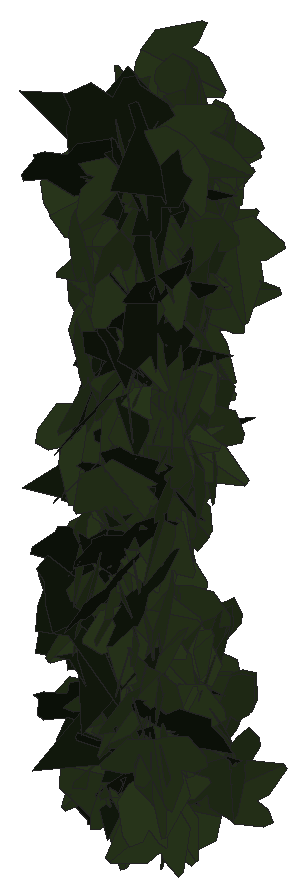
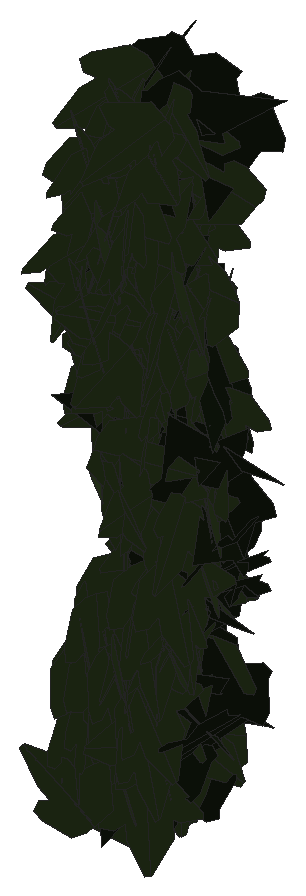
# SketchUp Ruby script. Lengths in inches.
U = 1.inch
M = Sketchup.active_model
def pt(a) = Geom::Point3d.new(a.map { |v| v * U })
def face(e, loops, mat)
  f = e.add_face(loops[0].map { |a| pt(a) })
  loops[1..].each { |l| e.add_face(l.map { |a| pt(a) }).erase! }
  f.material = f.back_material = mat if mat
  f
end
# faces: each face lists its corners as indices into pts; further lists are holes
def faces(e, pts, list, mat = nil) = list.each { |f| face(e, (f[0].is_a?(Array) ? f : [f]).map { |l| l.map { |i| pts[i] } }, mat) }
# xy, xz, yz: faces in a plane at the given z, y or x. An outline is a flat list of corners, or four numbers for a rectangle; further outlines are holes
def ring(l) = l.size == 4 ? [[l[0], l[1]], [l[2], l[1]], [l[2], l[3]], [l[0], l[3]]] : l.each_slice(2).to_a
def flat(e, list, mat, &to3) = list.each { |f| face(e, (f[0].is_a?(Array) ? f : [f]).map { |l| ring(l).map { |u, v| to3.(u, v) } }, mat) }
def xy(e, z, list, mat = nil) = flat(e, list, mat) { |x, y| [x, y, z] }
def xz(e, y, list, mat = nil) = flat(e, list, mat) { |x, z| [x, y, z] }
def yz(e, x, list, mat = nil) = flat(e, list, mat) { |y, z| [x, y, z] }
def lines(e, pts, list) = list.each { |a, b| e.add_line(pt(pts[a]), pt(pts[b])) }
# prism: a flat outline (further loops are holes) pulled along v
def prism(e, loops, v, mat = nil)
  f = face(e, loops, mat); d = Geom::Vector3d.new(v.map { |x| x * U })
  f.pushpull(f.normal.samedirection?(d) ? d.length : -d.length)
end
def box(e, o, s, mat = nil) = prism(e, [[o, [o[0] + s[0], o[1], o[2]], [o[0] + s[0], o[1] + s[1], o[2]], [o[0], o[1] + s[1], o[2]]]], [0, 0, s[2]], mat)
def at(x, y, z, deg = 0) = Geom::Transformation.translation(pt([x, y, z])) * Geom::Transformation.rotation(ORIGIN, Z_AXIS, deg.degrees)
def axes(o, x, y, z) = Geom::Transformation.new([*x, 0, *y, 0, *z, 0, *pt(o).to_a, 1])
def part(name) = M.definitions.add(name)
# library, detail: a bought-in or finely detailed component or shape, given as its bounding box
def library(name, o, s) = part(name).tap { |d| box(d.entities, o, s) }
def detail(e, o, s) = box(e.add_group.entities, o, s)
def put(e, d, t, mat = nil) = e.add_instance(d, t).tap { |i| i.material = mat if mat }
def group(e, t, mat = nil) = e.add_group.tap { |g| g.transformation = t; g.material = mat if mat }.entities
root = M.entities
M.materials.add("efeu1").color = [18, 25, 13]
M.materials.add("efeu2").color = [43, 57, 29]
c1 = part("ivyleaf_9")
p = [[1.54,2.16,1.25],[1.36,2.04,1.19],[-0.21,0.99,0.68],[-0.71,1.11,0.82],[-0.85,0.86,0.67],[-0.8,0.17,0.21],
  [-0.9,-0.01,0.1],[-0.67,-0.16,-0.02],[-0.08,-0.08,-0.05],[-0.03,-0.6,-0.4],[0.65,-0.88,-0.66],[0.83,-0.6,-0.49],
  [1.29,-0.42,-0.43],[1.8125,-0.07,-0.26],[1.21,0.44,0.15]]
faces(c1.entities,p,[[0,1,2,3,4,5,6,7,8,9,10,11,12,13,14]],"efeu1")
c2 = part("ivyleaf_10")
p = [[0,0.5,-0.03],[-0.0625,2.02,-0.43],[-0.19,2.01,-0.46],[-0.54,1.05,-0.29],[-0.52,0.625,-0.18],[-0.83,0.76,-0.28],
  [-1.16,0.64,-0.33],[-1.15,0.33,-0.24],[-0.77,-0.39,0.02],[-0.3,-0.51,0.16],[0.04,-0.48,0.23],[-0.02,2.01,-0.4375],
  [-0.06,2.01,-0.43],[0.04,-0.49,0.23],[0.67,-0.49,0.14],[1.38,0.36,-0.2],[1.375,0.51,-0.24],[0.81,0.65,-0.19],
  [0.62,0.59,-0.15],[0.6,1.09,-0.28],[0.5,1.23,-0.31]]
faces(c2.entities,p,[[0,1,2,3,4,5,6,7,8,9,10],[11,12,0,13,14,15,16,17,18,19,20]],"efeu2")
put(root,c1,axes([7.44,224.16,217.21],[0.0695,0.24852,0.36522],[0.0113,0.35407,-0.26258],[-0.46449,0.04579,0.04826]))
put(root,c2,axes([7.41,225.19,216.83],[-0.21146,-0.44477,0.0864],[0.0067,-0.09841,-0.49017],[0.45303,-0.20615,0.04758]))
put(root,c2,axes([7.5,224.99,216.29],[-0.41946,0.15413,0.12575],[-0.16369,-0.06633,-0.4184],[-0.13404,-0.40134,0.11744]))
put(root,c2,axes([7.34,225.65,222.36],[0.09342,0.35988,-0.23768],[-0.07488,-0.21822,-0.38466],[-0.45429,0.10997,0.01453]))
put(root,c2,axes([7.49,224.57,219.17],[0.1451,-0.14192,0.40417],[-0.25992,0.30555,0.20258],[-0.36345,-0.27517,0.01649]))
put(root,c2,axes([7.47,225.21,220.38],[-0.138,0.24686,0.34799],[-0.20383,0.27748,-0.28786],[-0.40015,-0.22648,0.02662]))
put(root,c1,axes([7.26,224.28,215.41],[0.36158,0.27576,0.03432],[0.02369,0.02527,-0.45106],[-0.29901,0.33547,0.00577]))
put(root,c2,axes([7.38,225.07,217.6],[-0.04548,-0.32229,-0.30066],[0.04105,0.28659,-0.33804],[0.46579,-0.05673,0.00043]))
put(root,c1,axes([7.24,224.46,218.98],[-0.04637,0.31707,0.30649],[0.02468,-0.29408,0.33251],[0.46685,0.04704,0.01286]))
put(root,c1,axes([7.41,224.06,222.36],[0.25403,0.35943,-0.07135],[-0.04654,-0.05378,-0.44669],[-0.39245,0.23904,0.00678]))
put(root,c2,axes([7.56,225.26,215.72],[-0.08941,0.18766,-0.39895],[-0.14836,0.35828,0.21311],[0.4367,0.16014,-0.00928]))
put(root,c2,axes([7.09,224.45,221.48],[0.26048,0.02603,-0.37552],[0.37507,0.10586,0.24919],[0.11039,-0.42112,0.03943]))
put(root,c2,axes([7.72,224.91,222.55],[-0.20705,0.0253,0.40524],[-0.41846,0.04151,-0.20107],[-0.0523,-0.43227,0.00441]))
put(root,c1,axes([7.75,224.73,222.38],[-0.14221,0.05193,0.42778],[-0.4477,-0.0093,-0.13679],[-0.00746,-0.43179,0.0544]))
put(root,c1,axes([7.24,224.39,217.02],[0.20606,-0.37128,-0.26399],[-0.10024,0.24568,-0.42378],[0.4444,0.22757,0.02681]))
put(root,c1,axes([7.4,224.73,217.9],[-0.22831,-0.16249,0.35745],[0.29444,0.2093,0.2773],[-0.28617,0.34499,0.00013]))
put(root,c2,axes([7.35,225.26,219.48],[-0.00836,-0.14836,-0.4252],[0.00132,-0.40892,0.1543],[-0.46972,0.00149,0.008]))
put(root,c2,axes([7.36,224.375,218.8],[0.46636,0.05248,0.00288],[0.00283,0.0014,-0.45239],[-0.05669,0.43182,0.00111]))
put(root,c2,axes([7.47,224.93,220.65],[0.19072,-0.462,0.01337],[-0.00066,-0.01474,-0.49978],[0.4622,0.19062,-0.00623]))
put(root,c1,axes([7.34,225,214.78],[-0.07854,-0.42886,-0.00358],[-0.0024,0.00386,-0.45238],[0.46318,-0.0727,-0.00295]))
put(root,c2,axes([7.125,224.6875,220.3125],[-0.06984,0.02546,-0.44659],[0.4094,-0.20188,-0.07182],[-0.2196,-0.38447,0.00814]))
put(root,c2,axes([7.33,224.51,217.5],[0.16124,-0.28835,0.30104],[0.19568,-0.22949,-0.33495],[0.3955,0.23111,0.04299]))
put(root,c2,axes([7.41,224.53,216.85],[0.23167,-0.4028,0.18462],[0.09254,-0.15975,-0.46467],[0.43332,0.24947,0.00053]))
put(root,c2,axes([7.66,224.72,214.6],[-0.20694,-0.20958,0.34271],[-0.17316,-0.29248,-0.29041],[0.38458,-0.24446,0.05365]))
put(root,c2,axes([7.4,224.51,220.15],[0.06217,0.36445,0.23963],[0.01198,0.23113,-0.38308],[-0.46551,0.05462,0.02214]))
put(root,c2,axes([7.33,225.74,222.8125],[0.10326,0.21905,0.378],[0.11473,0.34835,-0.24741],[-0.44372,0.14104,0.02399]))
put(root,c2,axes([7.6,224.89,217.43],[-0.19893,-0.39767,0.22866],[-0.0482,-0.22974,-0.44147],[0.45618,-0.19769,0.05307]))
put(root,c2,axes([7.53,224.49,219.35],[-0.04993,-0.47177,-0.15792],[0.02759,0.15585,-0.47429],[0.49673,-0.05608,0.01047]))
put(root,c1,axes([7.35,224.74,216.26],[0.09459,-0.37121,-0.21755],[-0.05448,0.20302,-0.39665],[0.45694,0.10105,-0.00226]))
put(root,c2,axes([7.56,225.43,216.25],[-0.04538,-0.49768,-0.01611],[-0.00701,0.01681,-0.49967],[0.49789,-0.04512,-0.0085]))
put(root,c1,axes([7.59,224.17,217.52],[0.21396,0.31324,-0.23683],[-0.12657,-0.1953,-0.38543],[-0.39864,0.23014,-0.00474]))
put(root,c2,axes([7.82,225.78,218.05],[-0.04942,0.07283,0.44347],[-0.44513,0.12289,-0.06782],[-0.14189,-0.41088,0.05832]))
put(root,c2,axes([7.48,224.22,221.39],[-0.08833,0.42319,0.06102],[-0.02101,0.05598,-0.44818],[-0.46094,-0.08365,0.00874]))
put(root,c2,axes([7.62,224.61,216.65],[0.17233,0.24853,-0.39816],[-0.23644,-0.32044,-0.30235],[-0.40546,0.29249,0.00708]))
put(root,c1,axes([7.86,224.63,218.32],[-0.40161,0.05547,0.22753],[-0.23896,-0.00631,-0.38945],[-0.04815,-0.4314,0.03496]))
put(root,c1,axes([7.68,224.09,219.19],[-0.03341,0.40681,0.15693],[-0.02049,0.14987,-0.42424],[-0.46816,-0.03559,0.00737]))
put(root,c2,axes([7.49,224.24,220.02],[-0.14157,0.41291,0.04096],[-0.01055,0.03822,-0.45054],[-0.44784,-0.13143,-0.00233]))
put(root,c2,axes([7.59,225.46,214.97],[-0.05436,-0.49657,0.02142],[0.00379,-0.02196,-0.4995],[0.49702,-0.05414,0.00615]))
put(root,c2,axes([7.55,225,220.04],[0.01472,-0.38608,-0.31737],[0.05253,0.31694,-0.38313],[0.49701,-0.02206,0.0499]))
put(root,c2,axes([7.6,224.36,217.4],[0.25313,-0.40183,-0.15638],[-0.05043,0.1525,-0.4735],[0.42823,0.25549,0.03668]))
put(root,c2,axes([7.63,225.4,215.31],[-0.09345,-0.47112,0.13897],[-0.03445,-0.13483,-0.48024],[0.48998,-0.09933,-0.00727]))
put(root,c1,axes([7.33,224.45,216.66],[0.0167,-0.42394,-0.10007],[0.10497,0.09722,-0.42922],[0.45762,-0.00682,0.1021]))
put(root,c2,axes([7.58,224.38,215.48],[-0.45029,-0.11766,-0.04092],[0.03968,0.01467,-0.45053],[0.12798,-0.41853,-0.00429]))
put(root,c2,axes([7.625,225.54,217.91],[0.06634,-0.04129,0.4458],[-0.17341,0.39958,0.06396],[-0.43155,-0.16691,0.04283]))
put(root,c2,axes([7.66,225.26,216.76],[-0.31347,-0.37297,0.1124],[-0.02551,-0.12431,-0.48363],[0.3887,-0.30894,0.0589]))
put(root,c1,axes([7.39,224.48,216.375],[-0.04108,-0.41752,-0.12064],[0.09877,0.10609,-0.42831],[0.45746,-0.0604,0.08164]))
put(root,c1,axes([7.82,224.77,215.125],[-0.40096,-0.13395,0.1902],[-0.17824,-0.08087,-0.41004],[0.16784,-0.40589,0.01893]))
put(root,c2,axes([7.52,225.27,216.05],[0.00729,0.38209,-0.21612],[0.00178,-0.20786,-0.39741],[-0.46974,0.00514,-0.00486]))
put(root,c1,axes([7.72,224,218.53],[0.05355,0.37705,0.21963],[-0.04351,0.21567,-0.39064],[-0.46471,0.02326,0.06188]))
put(root,c2,axes([7.66,224.74,214.49],[-0.14499,-0.4111,0.04877],[-0.00459,-0.04793,-0.44962],[0.44684,-0.13388,0.01121]))
put(root,c2,axes([7.9375,224.55,218.84],[-0.14986,0.09842,0.41637],[-0.44045,0.02913,-0.15445],[-0.06524,-0.42272,0.0863]))
put(root,c2,axes([7.59,224.38,217.8],[-0.43244,0.16162,-0.05483],[0.05137,-0.02301,-0.44905],[-0.17627,-0.4032,0.00365]))
put(root,c2,axes([7.85,224.88,221.05],[-0.32058,0.24718,-0.29348],[-0.23943,0.16998,0.4047],[0.29984,0.40001,0.00938]))
put(root,c2,axes([7.58,224.86,215.96],[0.15332,-0.34496,0.23272],[0.08206,-0.21065,-0.38785],[0.43643,0.16079,-0.00883]))
put(root,c2,axes([7.68,224.49,220.97],[-0.34202,-0.29707,-0.02725],[0.02097,0.01761,-0.45158],[0.3214,-0.31728,0.00046]))
put(root,c2,axes([7.58,224.93,215.78],[-0.10661,0.44521,-0.20106],[0.00213,-0.20537,-0.45587],[-0.4885,-0.09806,0.0419]))
put(root,c2,axes([7.75,224.65,222.09],[-0.32286,-0.3013,0.09906],[-0.06931,-0.07049,-0.4414],[0.33417,-0.30573,0.00416]))
put(root,c2,axes([7.89,224.61,214.67],[-0.32816,0.16436,-0.27493],[-0.26349,0.1037,0.35869],[0.2088,0.38918,0.02054]))
put(root,c2,axes([7.7,224.55,216.44],[-0.3194,-0.31901,0.00026],[0.00313,-0.00302,-0.45238],[0.34451,-0.29572,0.00434]))
put(root,c2,axes([7.51,225.03,219.8],[0.31288,-0.31824,0.22546],[0.16849,-0.15038,-0.44609],[0.35173,0.35512,0.01313]))
put(root,c2,axes([7.74,225.27,214.03],[-0.39056,-0.23756,0.04663],[-0.0161,-0.0586,-0.44801],[0.2606,-0.35966,0.0422]))
put(root,c1,axes([7.99,224.95,216.6],[-0.41894,0.04113,0.20022],[-0.20892,-0.00064,-0.40521],[-0.03948,-0.43305,0.01961]))
put(root,c2,axes([7.66,225.8125,221.3125],[-0.13904,0.40764,-0.0837],[-0.03334,-0.09341,-0.44068],[-0.44751,-0.11969,0.05884]))
put(root,c2,axes([7.8,225.04,218.32],[-0.29004,-0.37827,0.15096],[-0.04468,-0.15465,-0.47338],[0.40482,-0.28808,0.05591]))
put(root,c2,axes([7.91,224.51,222.09],[-0.25465,-0.22319,0.30109],[-0.19018,-0.23256,-0.33561],[0.34597,-0.29211,0.03713]))
put(root,c2,axes([7.93,224.51,219.33],[-0.07868,0.18574,0.40201],[-0.32999,0.25265,-0.18615],[-0.32501,-0.30149,0.09167]))
put(root,c2,axes([7.98,225.49,218.41],[0.13145,0.05643,-0.43035],[-0.41042,-0.16378,-0.13948],[-0.18705,0.39902,0.00361]))
put(root,c2,axes([7.74,224.96,221],[-0.34795,-0.28548,-0.06521],[0.05065,0.04161,-0.44768],[0.31158,-0.32557,-0.00004]))
put(root,c2,axes([7.71,224.7,214.18],[0.17443,0.40343,-0.02038],[-0.07242,0.00597,-0.44695],[-0.43016,0.16258,0.06699]))
put(root,c2,axes([7.67,225.3,214.74],[0.04119,-0.13513,0.42819],[0.00651,0.41343,0.14054],[-0.46795,-0.00614,0.03965]))
put(root,c1,axes([7.89,224.09,217.06],[-0.04819,0.42951,0.05455],[0.00387,0.05309,-0.449],[-0.46731,-0.04385,-0.00934]))
put(root,c2,axes([7.87,224.99,217.9375],[-0.42491,-0.17136,0.07408],[-0.07623,-0.01625,-0.44609],[0.18536,-0.3995,-0.01363]))
put(root,c2,axes([7.65,224.67,221.16],[0.12807,0.39994,0.12825],[0.03591,0.11877,-0.43384],[-0.45058,0.12314,0.00188]))
put(root,c2,axes([7.76,225.32,216.28],[0.13454,-0.43402,-0.20862],[0.03954,0.22583,-0.44434],[0.47993,0.10307,0.09509]))
put(root,c2,axes([7.4,224.34,214.53],[-0.04388,-0.02433,-0.49748],[0.49449,0.05767,-0.04644],[0.05964,-0.49607,0.019]))
put(root,c2,axes([7.82,224.7,222.45],[-0.29394,-0.33763,-0.03542],[0.0252,0.02493,-0.451],[0.36562,-0.27315,0.00261]))
put(root,c2,axes([7.68,224.89,219.85],[0.1725,0.40166,0.05078],[0.01905,0.04554,-0.44954],[-0.43657,0.1607,0.00045]))
put(root,c1,axes([8.11,224.5,215.09],[-0.26667,0.31186,0.18311],[-0.19027,0.08042,-0.40509],[-0.33674,-0.29241,0.08388]))
put(root,c1,axes([7.62,224.72,213.75],[0.44328,0.08739,0.11915],[-0.12119,-0.02312,0.43643],[0.09763,-0.4255,0.00076]))
put(root,c2,axes([7.75,224.41,216.54],[-0.05396,-0.15474,-0.4196],[0.10514,0.39168,-0.16877],[0.45469,-0.10893,-0.01077]))
put(root,c1,axes([7.69,224.46,220.3],[0.34132,-0.18724,-0.31375],[-0.24034,0.20833,-0.38579],[0.2752,0.41417,0.05221]))
put(root,c2,axes([7.76,224.9,218.82],[0.04793,-0.4431,-0.22663],[0.08265,0.23161,-0.43535],[0.49079,0.00427,0.09545]))
put(root,c2,axes([7.72,224.58,220.2],[-0.41279,-0.13935,-0.16018],[0.16234,0.03703,-0.42278],[0.15481,-0.41041,0.01625]))
put(root,c2,axes([7.73,224.74,217.51],[0.34987,0.2881,-0.0371],[-0.02866,-0.02384,-0.45088],[-0.31222,0.32504,-0.00018]))
put(root,c2,axes([7.68,225.12,214.65],[0.27324,-0.29888,0.19702],[0.15757,-0.12406,-0.4062],[0.34817,0.2907,0.02921]))
put(root,c2,axes([7.88,224.42,216.24],[0.28086,-0.32848,-0.12173],[-0.07338,0.09548,-0.43567],[0.36939,0.26872,0.00601]))
put(root,c1,axes([7.84,224.43,216.47],[-0.37507,-0.2335,-0.12348],[0.10645,0.06619,-0.43522],[0.26211,-0.361,0.00007]))
put(root,c1,axes([7.6,224.72,214.54],[0.45867,0.07796,0.05485],[0.04808,0.0484,-0.4472],[-0.08957,0.42521,0.04085]))
put(root,c2,axes([7.86,224.47,222.59],[-0.22221,0.37042,0.10234],[-0.06387,0.07966,-0.44048],[-0.40897,-0.21371,0.01319]))
put(root,c1,axes([7.77,224.87,218.61],[0.266,0.25092,0.26638],[-0.23069,-0.1469,0.36328],[0.31103,-0.32355,0.04164]))
put(root,c2,axes([8.1,224.25,216.53],[-0.0347,0.03985,-0.44926],[-0.27871,0.34643,0.0532],[0.3766,0.26005,-0.00202]))
put(root,c2,axes([7.85,224.5,219.62],[-0.09512,-0.31221,-0.30141],[0.0797,0.28029,-0.33734],[0.45311,-0.11484,-0.00393]))
put(root,c2,axes([7.85,225.5,221.43],[-0.42612,0.17068,-0.06916],[0.04557,-0.06898,-0.44451],[-0.19251,-0.39413,0.04785]))
put(root,c2,axes([7.875,225.47,222.8125],[0.38779,-0.23516,-0.07352],[-0.04483,0.0653,-0.44519],[0.26138,0.36009,0.03272]))
put(root,c2,axes([7.83,225.54,221.65],[-0.42186,-0.15801,-0.11242],[0.12443,0.00216,-0.43624],[0.16513,-0.40528,0.04151]))
put(root,c2,axes([7.76,225.59,222.76],[0.41168,-0.18582,0.10078],[0.0973,-0.0363,-0.44098],[0.20435,0.39163,0.00694]))
put(root,c2,axes([7.89,224.8,214.6],[-0.13579,-0.39723,-0.12999],[0.0509,0.11615,-0.43321],[0.44686,-0.13394,0.00984]))
put(root,c2,axes([7.94,224.99,219.66],[-0.10691,-0.48469,0.0604],[-0.01373,-0.05883,-0.49634],[0.48824,-0.10778,-0.00073]))
put(root,c2,axes([7.73,225.8,219.79],[-0.39484,0.04099,-0.24142],[0.24153,-0.07512,-0.38009],[-0.08049,-0.4265,0.04374]))
put(root,c2,axes([7.91,224.84,216.67],[-0.19934,0.39913,0.22574],[-0.08184,0.21123,-0.44574],[-0.45118,-0.21466,-0.01888]))
put(root,c2,axes([8.03,224.74,215.02],[-0.24599,-0.32557,0.18415],[-0.10465,-0.14829,-0.41319],[0.38633,-0.24747,0.00533]))
put(root,c2,axes([7.96,225.13,218.71],[-0.20138,-0.43407,0.14503],[-0.00156,-0.1578,-0.47445],[0.45765,-0.19154,0.0622]))
put(root,c2,axes([7.64,225.18,215.875],[0.36222,0.09612,0.2702],[0.26476,0.08699,-0.3626],[-0.13932,0.41523,0.01342]))
put(root,c2,axes([7.86,225.58,221.79],[0.33192,0.30361,-0.05295],[-0.04558,-0.02971,-0.4492],[-0.32934,0.3101,0.0088]))
put(root,c1,axes([7.82,224.83,219.86],[-0.16743,-0.39297,-0.10791],[0.04309,0.0958,-0.43934],[0.43683,-0.16007,0.00198]))
put(root,c2,axes([8,224.73,219.38],[-0.1397,-0.3801,0.29327],[-0.03472,-0.29663,-0.401],[0.47883,-0.1324,0.05649]))
put(root,c2,axes([7.82,225.6,220.13],[0.01737,-0.19938,0.40173],[0.03848,0.38585,0.20559],[-0.4679,0.02433,0.03182]))
put(root,c2,axes([7.99,225.32,215.07],[-0.22175,-0.40898,0.18321],[-0.01586,-0.19712,-0.45923],[0.44786,-0.20948,0.07445]))
put(root,c1,axes([7.77,224.77,220.41],[0.36968,-0.25347,-0.0919],[0.07677,-0.0525,0.44297],[-0.27956,-0.3496,0.00011]))
put(root,c1,axes([7.67,224.61,214.51],[0.46416,0.0672,-0.00033],[-0.00036,0.00417,0.45238],[0.07258,-0.42976,0.00433]))
put(root,c2,axes([7.93,224.77,215.49],[0.00875,-0.25261,0.3682],[0.04534,-0.352,-0.2622],[0.46753,0.03886,0.01854]))
put(root,c2,axes([7.99,224.88,221.03],[-0.29549,-0.3916,0.09661],[0.00728,-0.12492,-0.48409],[0.40328,-0.28468,0.07952]))
put(root,c2,axes([7.84,224.92,222.05],[0.26622,0.35791,0.01971],[0.01118,0.01588,-0.45197],[-0.38693,0.24672,0.0005]))
put(root,c2,axes([8,225.0625,219.42],[-0.19904,-0.42621,0.16949],[-0.00481,-0.18281,-0.46536],[0.45865,-0.18688,0.06867]))
put(root,c2,axes([8,225.49,215.65],[-0.0376,-0.49205,0.08047],[-0.0123,-0.07976,-0.49344],[0.49843,-0.03909,-0.00611]))
put(root,c2,axes([8.25,225.29,213.82],[-0.06542,-0.02097,-0.44746],[-0.43905,-0.14089,0.06667],[-0.15384,0.41102,0.00002]))
put(root,c1,axes([7.74,224.43,223],[-0.16748,-0.1878,-0.37485],[0.26513,0.26416,-0.25299],[0.34981,-0.29013,0.01229]))
put(root,c2,axes([7.85,224.53,217.83],[0.37158,0.24039,-0.11888],[0.0996,0.06758,0.43649],[0.26967,-0.35619,0.00259]))
put(root,c2,axes([7.91,224.83,220.13],[0.13423,0.40739,-0.09189],[-0.04375,-0.07996,-0.44269],[-0.44808,0.12985,0.0157]))
put(root,c2,axes([7.88,225.62,220.5],[-0.14604,0.40013,-0.10827],[0.04329,-0.09633,-0.43919],[-0.44442,-0.14086,-0.0072]))
put(root,c2,axes([8.02,224.47,215.39],[0.32153,-0.2873,-0.13973],[-0.09327,0.10389,-0.43003],[0.3296,0.30966,0.01463]))
put(root,c1,axes([7.83,224.5,222.41],[0.3518,-0.20067,-0.21528],[-0.17995,0.12384,-0.39755],[0.25409,0.36554,0.0165]))
put(root,c2,axes([7.96,225,219.32],[0.08274,-0.31766,0.29863],[-0.08187,0.27703,0.33977],[-0.45515,-0.10758,-0.00683]))
put(root,c2,axes([7.88,224.88,216.79],[0.04084,-0.24646,0.37071],[0.16522,-0.32718,-0.25214],[0.43789,0.14643,0.06056]))
put(root,c2,axes([7.98,225.68,221.47],[0.16687,-0.40293,0.05698],[0.02678,-0.04916,-0.44876],[0.43835,0.15639,0.00573]))
put(root,c2,axes([7.88,225.64,220.8],[0.13454,-0.40707,-0.09301],[0.02667,-0.08597,0.44273],[-0.44933,-0.12699,-0.00157]))
put(root,c2,axes([8.12,225.36,215.79],[0.23067,-0.26317,-0.28358],[-0.17681,0.21821,-0.35239],[0.36911,0.26898,0.00842]))
put(root,c2,axes([7.96,225.59,222.2],[-0.13095,0.32234,0.27637],[0.10157,-0.24854,0.35817],[0.4396,0.15345,-0.00043]))
put(root,c2,axes([7.99,225.26,215.86],[0.12877,-0.44891,0.1786],[0.03586,-0.17544,-0.46683],[0.4818,0.13304,-0.01299]))
put(root,c2,axes([7.98,224.44,215.625],[-0.28532,0.34532,0.01419],[-0.00948,0.01047,-0.45218],[-0.37311,-0.26433,0.00063]))
put(root,c2,axes([7.9375,225.04,219.34],[-0.0118,-0.40106,-0.17482],[-0.00677,-0.16799,0.41725],[-0.4696,0.0125,-0.00162]))
put(root,c2,axes([7.91,224.8,214.65],[0.25713,0.35394,0.08868],[0.0087,0.09674,-0.44099],[-0.39309,0.23366,0.04825]))
put(root,c2,axes([8.09,225.07,215.87],[-0.09013,0.18303,0.40112],[-0.18284,0.34659,-0.20914],[-0.42327,-0.18869,0.00493]))
put(root,c2,axes([7.88,224.65,215.47],[0.15076,0.22557,0.35854],[0.05242,0.35247,-0.26028],[-0.44186,0.11878,0.09146]))
put(root,c1,axes([8.08,224.18,217.74],[0.13028,0.41206,-0.07262],[-0.02825,-0.06509,-0.44648],[-0.45049,0.12325,0.007]))
put(root,c2,axes([7.94,225.35,219.18],[0.25984,0.35898,-0.05171],[-0.02734,-0.04288,-0.44943],[-0.39045,0.2419,-0.00294]))
put(root,c2,axes([7.83,225.6,220.01],[0.14541,0.17235,-0.39106],[0.25188,0.29496,0.22745],[0.36895,-0.26929,-0.00115]))
put(root,c2,axes([7.89,224.24,218.4],[-0.32727,-0.21274,-0.23747],[0.22614,0.09741,-0.38338],[0.24993,-0.36671,0.03592]))
put(root,c2,axes([8.13,224.97,218.97],[-0.30117,-0.31864,0.10363],[-0.07095,-0.07493,-0.44037],[0.35352,-0.28649,-0.00009]))
put(root,c2,axes([8.13,224.76,216.1],[-0.45359,0.04967,0.10586],[-0.11127,-0.00516,-0.43949],[-0.05081,-0.43212,0.01742]))
put(root,c2,axes([7.97,224.9,217.06],[0.19607,0.38063,-0.111],[-0.04158,-0.09986,-0.43849],[-0.4249,0.18541,-0.00831]))
put(root,c2,axes([8.08,224.7,217.8125],[0.43389,0.05466,-0.16388],[-0.16887,-0.01961,-0.42167],[-0.0627,0.43111,0.0016]))
put(root,c2,axes([8.12,225.43,215.58],[-0.38188,-0.28888,0.14393],[-0.04631,-0.17162,-0.46733],[0.31941,-0.37026,0.10433]))
put(root,c1,axes([7.73,224.86,218.52],[0.171,0.31202,-0.26879],[0.12991,0.22877,0.36388],[0.41784,-0.19882,-0.00313]))
put(root,c2,axes([8.06,224.76,222.08],[0.32205,-0.3255,-0.20083],[-0.04971,0.22469,-0.4439],[0.37923,0.30588,0.11236]))
put(root,c1,axes([8.33,224.26,217.08],[-0.24022,0.38628,0.20756],[-0.11972,0.1699,-0.45475],[-0.42186,-0.26818,0.01086]))
put(root,c1,axes([7.8125,224.28,218.49],[0.43107,0.14312,0.10099],[0.09768,0.03545,-0.44098],[-0.15921,0.40925,0.00288]))
put(root,c1,axes([7.99,224.8125,221.78],[0.37797,0.32731,0.00307],[-0.06377,0.07823,-0.48971],[-0.32105,0.3698,0.10088]))
put(root,c2,axes([8.2,224.96,214.84],[-0.25589,0.33635,0.14692],[-0.22718,0.01167,-0.39581],[-0.3219,-0.27561,0.16254]))
put(root,c2,axes([8.14,224.71,220.9],[0.1079,0.00584,-0.44026],[-0.08313,0.42796,-0.01275],[0.44962,0.07772,0.1033]))
put(root,c2,axes([7.94,224.82,220.8],[0.00913,-0.29726,-0.33017],[0.05417,-0.31475,0.30789],[-0.46658,-0.04236,0.02929]))
put(root,c2,axes([8,225.63,221.35],[-0.12605,0.41869,0.01812],[-0.00472,0.01687,-0.45204],[-0.45255,-0.11679,-0.00033]))
put(root,c2,axes([8.375,224.92,219.46],[-0.04728,0.01177,0.44994],[-0.45053,0.11466,-0.04714],[-0.12448,-0.41945,-0.00026]))
put(root,c2,axes([7.78,224.42,217.71],[0.32663,0.09814,0.30874],[0.29045,0.12901,-0.3293],[-0.17223,0.40367,0.03019]))
put(root,c2,axes([8.0625,225.16,217.53],[0.26206,-0.39873,-0.14946],[0.01216,0.18243,-0.46537],[0.42565,0.24027,0.10532]))
put(root,c2,axes([8.25,224.72,220.84],[0.21927,0.00585,0.40006],[-0.32561,0.2726,0.16118],[-0.25809,-0.33894,0.13654]))
put(root,c2,axes([8.33,224.83,219.53],[0.19914,0.06803,-0.40359],[-0.40777,-0.09191,-0.20333],[-0.12158,0.4197,0.02089]))
put(root,c2,axes([8.03,224.63,221.72],[-0.19865,0.39393,0.01511],[-0.00508,0.01384,-0.45214],[-0.42571,-0.18399,-0.00166]))
put(root,c2,axes([8,224.41,216.46],[0.41163,0.20925,-0.01379],[-0.01724,0.00152,-0.45209],[-0.22578,0.38136,0.00937]))
put(root,c2,axes([8.21,224.55,215.34],[-0.15122,0.34448,0.23476],[-0.23759,0.139,-0.36252],[-0.37603,-0.22636,0.13465]))
put(root,c2,axes([7.99,224.8125,217.71],[0.10398,0.4216,0.04889],[0.01202,0.04568,-0.44975],[-0.45799,0.09692,-0.00071]))
put(root,c2,axes([8.125,224.39,215.62],[0.02287,-0.43407,0.01973],[0.00205,-0.0189,-0.45197],[0.46924,0.02124,0.00101]))
put(root,c2,axes([8.17,225.08,216.6],[-0.43667,-0.15896,0.02281],[-0.02086,-0.0108,-0.45181],[0.17205,-0.40477,0.0031]))
put(root,c2,axes([8.29,224.3,216],[-0.43352,-0.03102,0.17131],[-0.17598,-0.02798,-0.41845],[0.04243,-0.43299,0.01477]))
put(root,c1,axes([8.13,224.61,215.49],[0.23223,0.37744,-0.02397],[-0.01851,-0.01676,-0.45171],[-0.40797,0.21561,0.00685]))
put(root,c2,axes([8.2,224.5,215.4375],[0.44002,0.05315,0.14856],[-0.15389,-0.01183,0.42726],[0.05841,-0.43158,0.00658]))
put(root,c2,axes([8.11,225.05,215.83],[-0.31442,0.32306,-0.01055],[0.0067,-0.00806,-0.45228],[-0.34901,-0.2912,0.00082]))
put(root,c2,axes([8.14,225.8,220.46],[0.23247,-0.37788,0.01048],[0.00837,-0.00718,-0.45227],[0.40817,0.21536,0.00331]))
put(root,c2,axes([8.2,225.14,214.84],[-0.45652,-0.10223,0.01009],[-0.01023,-0.0021,-0.45229],[0.11043,-0.42281,-0.00019]))
put(root,c2,axes([8.11,225.125,214.14],[0.22886,-0.36544,0.10795],[0.06239,-0.08648,-0.43928],[0.40552,0.21954,0.00666]))
put(root,c2,axes([7.79,224.89,220.79],[-0.09497,-0.00941,-0.49081],[0.48863,0.0462,-0.09544],[0.04715,-0.49777,0.00042]))
put(root,c2,axes([8.15,225.12,220.6875],[0.01899,0.36317,-0.24834],[-0.09111,-0.23159,-0.37277],[-0.46049,0.0608,0.06351]))
put(root,c1,axes([7.8,224.32,219.81],[0.22054,0.04072,0.39721],[0.40669,0.06398,-0.21648],[-0.08171,0.42834,-0.00542]))
put(root,c2,axes([8.17,225.65,221.48],[0.00324,0.40378,0.16828],[-0.10902,0.15804,-0.4082],[-0.45697,-0.03484,0.09858]))
put(root,c2,axes([8.17,224.74,222.1875],[0.09932,0.46385,-0.15805],[-0.12509,-0.13192,-0.46578],[-0.4738,0.13207,0.08984]))
put(root,c2,axes([8.32,224.52,214.14],[0.37489,-0.03183,-0.27064],[-0.27951,0.02737,-0.36251],[0.04523,0.43297,0.00302]))
put(root,c2,axes([8.26,224.81,220.04],[0.27929,-0.26806,-0.2337],[-0.15083,0.17709,-0.38685],[0.34635,0.29328,0.01998]))
put(root,c2,axes([8.22,224.95,219.41],[0.13819,-0.42151,-0.23073],[-0.04693,0.22709,-0.44297],[0.47823,0.14409,0.02321]))
put(root,c2,axes([8.17,224.09,221.63],[-0.08652,-0.32809,-0.28512],[0.05844,0.2689,-0.35113],[0.45805,-0.09628,-0.00906]))
put(root,c2,axes([8.07,224.24,220.88],[0.20237,0.38811,0.06136],[0.02679,0.05355,-0.44822],[-0.42313,0.18901,0.00097]))
put(root,c1,axes([8.51,224.25,222.08],[-0.11974,0.14926,0.40899],[-0.31371,0.26699,-0.19055],[-0.32858,-0.3093,0.03289]))
put(root,c2,axes([8.1875,224.49,222.27],[-0.11351,0.34898,0.24697],[-0.0861,0.2239,-0.3789],[-0.44768,-0.13155,0.01025]))
put(root,c1,axes([8.18,224.7,214.56],[0.24265,0.43715,0.00473],[0.00237,0.0041,-0.49998],[-0.43717,0.24266,-0.00008]))
put(root,c2,axes([8.17,224.79,222.03],[0.13171,-0.45036,0.17271],[0.03702,-0.16906,-0.46909],[0.48092,0.13635,-0.01119]))
put(root,c2,axes([7.93,224.79,216.41],[0.38494,0.11914,0.22784],[0.22422,0.06994,-0.39084],[-0.1492,0.41248,0.00047]))
put(root,c2,axes([8.14,225.72,220.78],[0.01753,0.34647,0.27303],[-0.02804,0.26302,-0.35932],[-0.46863,-0.00278,0.03171]))
put(root,c2,axes([8.15,225.62,222.11],[-0.34228,-0.26972,-0.13168],[0.12759,0.05596,-0.43149],[0.29543,-0.33666,0.03378]))
put(root,c2,axes([8.12,224.41,217.16],[-0.20306,0.3743,-0.12204],[0.05645,-0.10507,-0.43563],[-0.41987,-0.19515,0.00046]))
put(root,c2,axes([8.4,225.07,219.97],[-0.36019,0.17258,0.22835],[-0.24977,0.02104,-0.38254],[-0.16908,-0.39874,0.07865]))
put(root,c2,axes([8.35,224.59,219.99],[0.35126,-0.24897,-0.25423],[-0.20086,0.15614,-0.43044],[0.29372,0.40452,0.00968]))
put(root,c2,axes([8.23,224.76,215.28],[-0.00867,0.01815,0.45193],[0.05138,-0.43198,0.01968],[0.4669,0.04787,0.00623]))
put(root,c2,axes([8.15,224.89,220.12],[-0.0869,0.35095,-0.25387],[0.02351,-0.2447,-0.37335],[-0.46109,-0.07862,0.02881]))
put(root,c2,axes([8.28,225.39,216.16],[-0.11162,-0.4849,-0.04914],[0.00598,0.04905,-0.49755],[0.48734,-0.11166,-0.00515]))
put(root,c2,axes([8.14,224.88,219.31],[-0.2712,0.31078,-0.17888],[0.0912,-0.15237,-0.41454],[-0.37262,-0.26349,0.02874]))
put(root,c2,axes([8.18,224.77,222.1],[0.15413,0.46686,-0.09101],[-0.02446,-0.08777,-0.49163],[-0.47502,0.156,-0.00422]))
put(root,c2,axes([8.5,224.85,215.84],[0.1521,0.10012,0.41518],[-0.34077,-0.24465,0.17957],[0.2854,-0.34547,-0.00685]))
put(root,c2,axes([8.29,224.6875,215.36],[-0.04432,-0.43304,-0.00473],[0.00078,0.0045,-0.45238],[0.4677,-0.04104,0.0003]))
put(root,c2,axes([8.38,224.92,219.78],[0.39703,-0.01857,-0.24108],[-0.25007,0.0111,-0.38281],[0.02336,0.43446,-0.00052]))
put(root,c2,axes([8.18,225.0625,221.67],[-0.32234,-0.24176,-0.21237],[0.16541,0.13528,-0.39938],[0.29908,-0.33538,-0.00801]))
put(root,c2,axes([8.19,224.63,217.64],[0.49594,-0.06337,0.00517],[0.00506,-0.00119,-0.49997],[0.06338,0.49597,-0.00054]))
put(root,c2,axes([8.24,225.61,222.07],[0.06179,0.4295,-0.04006],[-0.05462,-0.03191,-0.44811],[-0.46251,0.06115,0.04756]))
put(root,c2,axes([8.4,224.64,215.02],[0.1708,-0.01631,0.4211],[-0.2649,0.34213,0.11396],[-0.34838,-0.26815,0.1198]))
put(root,c2,axes([8.61,224.4,218.98],[-0.15497,0.0396,0.42509],[-0.44346,-0.00793,-0.14912],[-0.00605,-0.43312,0.04159]))
put(root,c2,axes([8.28,224.95,219.91],[0.26832,-0.40833,-0.10616],[0.00851,0.13103,-0.48245],[0.42182,0.25709,0.07726]))
put(root,c2,axes([8.32,224.95,218.04],[0.03405,-0.49408,0.06876],[0.01816,-0.06765,-0.49507],[0.49851,0.03621,0.01334]))
put(root,c2,axes([8.29,225.66,222.31],[0.36521,-0.27316,-0.01669],[-0.01349,0.01008,-0.45209],[0.29521,0.33839,-0.00001]))
put(root,c2,axes([8.46,225.11,218.61],[0.25964,-0.10644,-0.36042],[-0.21518,0.30861,-0.24231],[0.32711,0.2875,0.12668]))
put(root,c2,axes([8.5,224.32,221.18],[0.34203,-0.01556,-0.30972],[-0.31852,0.04793,-0.32879],[0.04766,0.43207,0.02532]))
put(root,c2,axes([8.37,224.83,220.78],[-0.43431,-0.16565,0.00859],[-0.00979,0.00031,-0.4523],[0.17886,-0.40222,-0.00388]))
put(root,c2,axes([7.98,225.72,220.13],[-0.12221,-0.11188,0.42104],[0.40038,0.1705,0.15677],[-0.21324,0.38424,0.05304]))
put(root,c1,axes([8.17,224.41,222.1875],[-0.28686,-0.08953,-0.34596],[0.34322,0.09845,-0.29146],[0.1436,-0.41415,0.00551]))
put(root,c2,axes([8.08,225.41,217.49],[-0.02088,-0.15203,-0.42339],[0.25772,-0.34429,0.12193],[-0.39224,-0.21812,0.10265]))
put(root,c2,axes([8.375,225,219.84],[0.31292,-0.31661,-0.07381],[-0.05304,0.05126,-0.44634],[0.34638,0.29387,-0.00167]))
put(root,c2,axes([8.05,224.47,219.07],[-0.10057,-0.13113,-0.42034],[0.41325,0.15405,-0.14366],[0.19956,-0.38509,0.08566]))
put(root,c2,axes([8.04,224.32,220.46],[0.29423,-0.00425,0.35266],[0.36617,-0.00583,-0.28336],[0.00778,0.43494,-0.00035]))
put(root,c2,axes([8.47,225.04,219],[-0.35591,-0.27165,0.08593],[-0.07038,-0.05085,-0.44416],[0.29847,-0.33592,-0.00226]))
put(root,c2,axes([8.35,224.79,219.34],[0.25749,-0.37506,-0.20744],[0.02389,0.25418,-0.42991],[0.42794,0.21148,0.14882]))
put(root,c2,axes([8.6875,225.01,215.18],[-0.14918,0.17527,-0.38834],[-0.36428,0.17867,0.21699],[0.25643,0.35578,0.08233]))
put(root,c2,axes([8.41,224.44,217.08],[0.36931,-0.32652,-0.0836],[-0.05808,0.06051,-0.49292],[0.33201,0.37379,0.00676]))
put(root,c2,axes([8.21,224.34,216.43],[0.26905,0.21966,0.29215],[0.13015,0.27066,-0.33125],[-0.36247,0.26023,0.09791]))
put(root,c2,axes([8.05,225.07,214.97],[0.00634,0.00647,-0.45231],[0.41345,-0.20656,0.00218],[-0.223,-0.38278,-0.00881]))
put(root,c1,axes([8.27,224.71,222.48],[0.22753,-0.27129,-0.35303],[0.21493,-0.28028,0.35391],[-0.38992,-0.3128,-0.01092]))
put(root,c2,axes([8.45,224.57,215.24],[-0.10175,0.39779,0.15465],[-0.1117,0.12624,-0.41935],[-0.44484,-0.12268,0.06993]))
put(root,c2,axes([8.21,224.77,215.97],[0.0662,-0.09903,0.43588],[0.30217,-0.31267,-0.11939],[0.35358,0.28575,0.02042]))
put(root,c2,axes([8.14,224.875,215.73],[0.34929,-0.07819,-0.2914],[0.28992,-0.0812,0.34582],[-0.12104,-0.42014,-0.0126]))
put(root,c2,axes([8.39,225.03,218.98],[-0.0464,0.12521,-0.43094],[-0.03009,-0.41634,-0.12783],[-0.46653,0.0144,0.0511]))
put(root,c2,axes([8.63,224.74,218.58],[0.1574,-0.05589,-0.42227],[-0.2484,0.34554,-0.13532],[0.36638,0.25827,0.08966]))
put(root,c2,axes([8.47,225.17,216.24],[-0.01026,-0.49889,0.03164],[0.00242,-0.03169,-0.49899],[0.49989,-0.01009,0.00307]))
put(root,c2,axes([8.46,225.3125,214.875],[0.00647,-0.46899,-0.17322],[0.02534,0.17332,-0.46832],[0.49932,-0.00272,0.02601]))
put(root,c2,axes([8.25,224.45,214.42],[0.22533,0.30882,0.2333],[0.13663,0.18525,-0.3876],[-0.38893,0.244,-0.001]))
put(root,c2,axes([8.42,224.66,218.15],[-0.07127,0.36501,-0.3342],[-0.04775,-0.34114,-0.36241],[-0.49259,-0.01974,0.08348]))
put(root,c2,axes([8.39,224.62,215.02],[0.10731,0.47813,-0.0994],[-0.034,-0.09421,-0.48987],[-0.48716,0.11189,0.0123]))
put(root,c2,axes([8.49,224.25,215.14],[-0.36901,-0.26696,-0.03622],[0.0306,0.0203,-0.45095],[0.28915,-0.34285,0.0015]))
put(root,c2,axes([8.42,225.05,222.24],[-0.01828,-0.39802,-0.18169],[0.10922,0.16643,-0.40453],[0.45656,-0.05575,0.0895]))
put(root,c2,axes([8.22,224.5,216.02],[0.15961,-0.35006,-0.22023],[0.21773,-0.1336,0.37603],[-0.38449,-0.22098,0.12152]))
put(root,c2,axes([8.51,224.84,221.42],[-0.31846,-0.31742,-0.0406],[0.0254,0.03144,-0.45055],[0.34446,-0.29578,-0.00431]))
put(root,c2,axes([8.54,225.35,215.47],[-0.15576,-0.45248,0.14492],[-0.0124,-0.14858,-0.47725],[0.47496,-0.15227,0.03507]))
put(root,c1,axes([8.56,224.34,215.57],[0.29228,0.25594,-0.23366],[-0.21367,-0.11544,-0.3846],[-0.29938,0.33226,0.04637]))
put(root,c2,axes([8.51,225.34,216.02],[0.22411,-0.44119,-0.07158],[-0.01944,0.07037,-0.49464],[0.44654,0.22449,0.01439]))
put(root,c2,axes([8.64,224.45,222.6],[0.38586,-0.01317,-0.25772],[-0.26598,0.03454,-0.37118],[0.03292,0.43343,0.02175]))
put(root,c2,axes([8.27,225.73,213.9],[-0.28722,-0.11078,0.33896],[0.32449,0.12632,0.29961],[-0.18145,0.40124,-0.00074]))
put(root,c2,axes([8.26,224.86,218.79],[-0.18854,-0.20026,-0.35822],[0.38764,0.08422,-0.24012],[0.18682,-0.37687,0.1367]))
put(root,c2,axes([8.51,224.54,215.64],[-0.35634,-0.27845,-0.05528],[0.11331,-0.04418,-0.43664],[0.28442,-0.33127,0.10469]))
put(root,c2,axes([8.61,225.24,215.5],[-0.14557,-0.45529,0.1467],[-0.01773,-0.1481,-0.47723],[0.47801,-0.14414,0.02697]))
put(root,c2,axes([8.51,224.31,221.54],[-0.14657,0.4092,0.06034],[-0.01882,0.05534,-0.44836],[-0.44595,-0.13682,-0.00091]))
put(root,c2,axes([8.625,224.94,219.39],[-0.06413,-0.41465,0.27195],[-0.03285,-0.27006,-0.41951],[0.49478,-0.07167,0.0074]))
put(root,c1,axes([8.51,224.14,220.27],[-0.08258,-0.15322,0.41587],[0.27263,0.31199,0.17453],[-0.37359,0.26155,0.03544]))
put(root,c2,axes([8.34,224.7,222.65],[-0.2438,-0.14354,-0.41226],[0.35261,0.21362,-0.2829],[0.25735,-0.42868,-0.00293]))
put(root,c1,axes([8.43,223.95,220.89],[0.22565,0.2314,0.31549],[0.19634,0.2437,-0.32355],[-0.36228,0.27621,0.02116]))
put(root,c2,axes([8.5,225.64,220.96],[0.08377,0.42795,-0.00841],[-0.00006,-0.00821,-0.45232],[-0.46227,0.07755,-0.00147]))
put(root,c2,axes([8.61,225.33,214.61],[-0.06562,-0.47576,-0.1391],[0.02042,0.1376,-0.48026],[0.49526,-0.06871,0.00137]))
put(root,c2,axes([8.64,224.91,220.98],[0.03637,-0.48602,-0.11162],[-0.00654,0.11144,-0.48738],[0.49863,0.03691,0.00174]))
